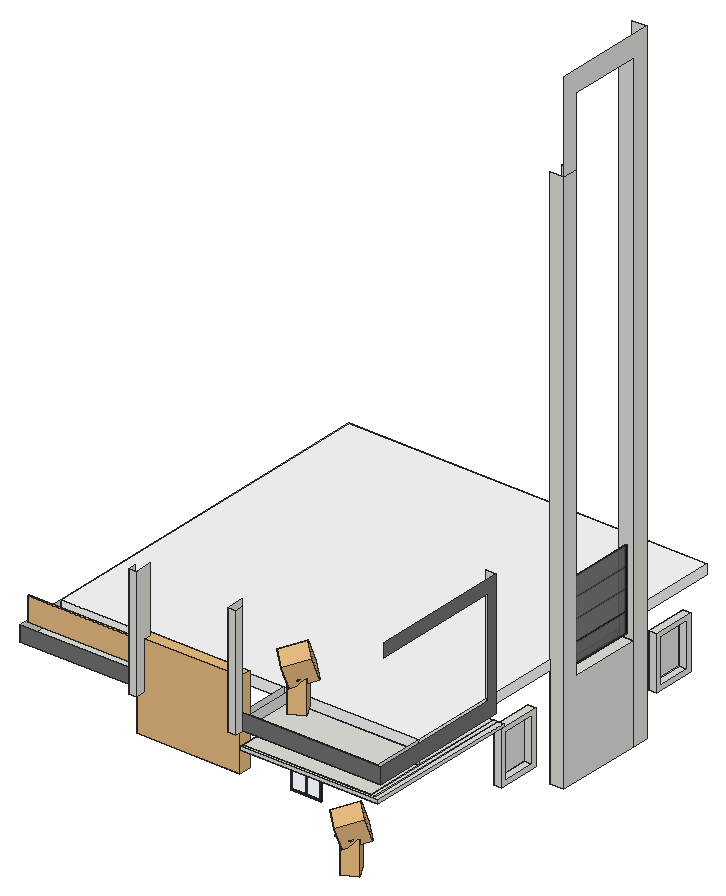
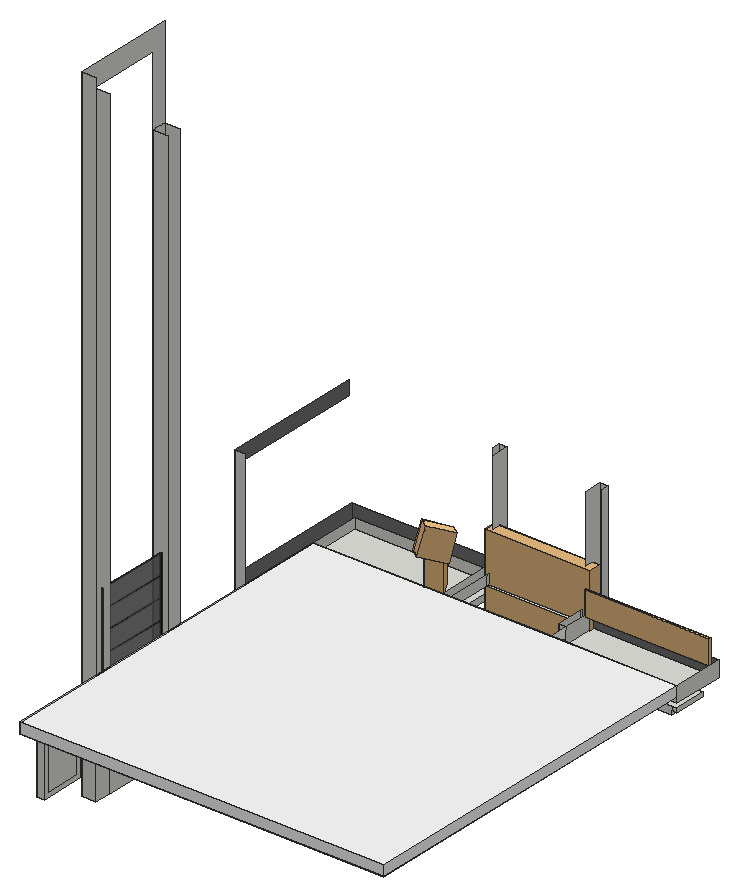
# SketchUp Ruby script. Lengths in inches.
U = 1.inch
M = Sketchup.active_model
def pt(a) = Geom::Point3d.new(a.map { |v| v * U })
def face(e, loops, mat)
  f = e.add_face(loops[0].map { |a| pt(a) })
  loops[1..].each { |l| e.add_face(l.map { |a| pt(a) }).erase! }
  f.material = f.back_material = mat if mat
  f
end
# faces: each face lists its corners as indices into pts; further lists are holes
def faces(e, pts, list, mat = nil) = list.each { |f| face(e, (f[0].is_a?(Array) ? f : [f]).map { |l| l.map { |i| pts[i] } }, mat) }
# xy, xz, yz: faces in a plane at the given z, y or x. An outline is a flat list of corners, or four numbers for a rectangle; further outlines are holes
def ring(l) = l.size == 4 ? [[l[0], l[1]], [l[2], l[1]], [l[2], l[3]], [l[0], l[3]]] : l.each_slice(2).to_a
def flat(e, list, mat, &to3) = list.each { |f| face(e, (f[0].is_a?(Array) ? f : [f]).map { |l| ring(l).map { |u, v| to3.(u, v) } }, mat) }
def xy(e, z, list, mat = nil) = flat(e, list, mat) { |x, y| [x, y, z] }
def xz(e, y, list, mat = nil) = flat(e, list, mat) { |x, z| [x, y, z] }
def yz(e, x, list, mat = nil) = flat(e, list, mat) { |y, z| [x, y, z] }
def lines(e, pts, list) = list.each { |a, b| e.add_line(pt(pts[a]), pt(pts[b])) }
# prism: a flat outline (further loops are holes) pulled along v
def prism(e, loops, v, mat = nil)
  f = face(e, loops, mat); d = Geom::Vector3d.new(v.map { |x| x * U })
  f.pushpull(f.normal.samedirection?(d) ? d.length : -d.length)
end
def box(e, o, s, mat = nil) = prism(e, [[o, [o[0] + s[0], o[1], o[2]], [o[0] + s[0], o[1] + s[1], o[2]], [o[0], o[1] + s[1], o[2]]]], [0, 0, s[2]], mat)
def at(x, y, z, deg = 0) = Geom::Transformation.translation(pt([x, y, z])) * Geom::Transformation.rotation(ORIGIN, Z_AXIS, deg.degrees)
def axes(o, x, y, z) = Geom::Transformation.new([*x, 0, *y, 0, *z, 0, *pt(o).to_a, 1])
def part(name) = M.definitions.add(name)
# library, detail: a bought-in or finely detailed component or shape, given as its bounding box
def library(name, o, s) = part(name).tap { |d| box(d.entities, o, s) }
def detail(e, o, s) = box(e.add_group.entities, o, s)
def put(e, d, t, mat = nil) = e.add_instance(d, t).tap { |i| i.material = mat if mat }
def group(e, t, mat = nil) = e.add_group.tap { |g| g.transformation = t; g.material = mat if mat }.entities
root = M.entities
M.materials.add("Material__1").color = [51, 42, 44]
M.materials.add("Material__2").color = [97, 132, 37]
M.materials.add("[0136_Charcoal]").color = [35, 35, 35]
M.materials.add("[Color M00]").color = [255, 255, 255]
M.materials.add("[Color M05]").color = [114, 114, 114]
M.materials.add("[Translucent_Glass_Blue]").color = [68, 104, 165]
M.materials["[Translucent_Glass_Blue]"].alpha = 0.07
M.materials.add("[Translucent_Glass_Green_Dark]").color = [33, 68, 103]
M.materials["[Translucent_Glass_Green_Dark]"].alpha = 0.08
M.materials.add("{045efeae-c101-a24d-bd9b-6f5600100adb}").color = [102, 102, 102]
M.materials["{045efeae-c101-a24d-bd9b-6f5600100adb}"].alpha = 0.7
M.materials.add("{16756a1b-d383-d94f-ad82-104813d2624f}").color = [19, 21, 27]
c1 = library("\#1",[-138.85,-135.75,0],[277.7,270.97,9.64])
c2 = library("\#2",[-34.84,-73.35,-33.91],[69.68,146.26,68.31])
c3 = library("\#5",[-4127.85,-1300.75,-2324.72],[5349.84,4521.24,5423.31])
c4 = part("\#3")
put(c4.entities,c3,at(450.18,-1111.4375,0),"Material__2")
c5 = part("12")
put(c5.entities,c1,axes([-49.79,-36.9375,349.64],[0.59279,0,0],[0,0.59279,0],[0,0,0.59279]),"Material__1")
put(c5.entities,c2,axes([-39.24,-18.18,177.19],[1.20819,-2.09264,0],[0,0,2.41638],[2.09264,1.20819,0]))
put(c5.entities,c4,axes([-83.44,-46.04,442.44],[-0.03636,-0.03293,-0.01473],[-0.00083,-0.02391,0.05549],[0.02997,-0.02791,-0.01158]))
c6 = part("Two-panel window \#1")
xy(c6.entities,-18,[[0,-31,2,35]],"[0136_Charcoal]")
xy(c6.entities,-16,[[0,-29,0.9375,33],[0.9375,-29,1.125,33],[1.125,-29,2,1],[1.125,3,2,33]],"[0136_Charcoal]")
xy(c6.entities,76,[[0,-29,0.9375,33],[0.9375,-29,1.125,33],[1.125,-29,2,1],[1.125,3,2,33]],"[0136_Charcoal]")
xy(c6.entities,78,[[0,-31,2,35]],"[0136_Charcoal]")
xz(c6.entities,-31,[[0,-18,2,78]],"[0136_Charcoal]")
xz(c6.entities,-29,[[0,-16,0.9375,76],[0.9375,-16,1.125,76],[1.125,-16,2,76]],"[0136_Charcoal]")
xz(c6.entities,1,[[1.125,-16,2,76]],"[0136_Charcoal]")
xz(c6.entities,3,[[1.125,-16,2,76]],"[0136_Charcoal]")
xz(c6.entities,33,[[0,-16,0.9375,76],[0.9375,-16,1.125,76],[1.125,-16,2,76]],"[0136_Charcoal]")
xz(c6.entities,35,[[0,-18,2,78]],"[0136_Charcoal]")
yz(c6.entities,0,[[[-31,-18,35,78],[-29,-16,33,76]]],"[0136_Charcoal]")
yz(c6.entities,0.9375,[[-29,-16,33,76]],"[Translucent_Glass_Blue]")
yz(c6.entities,1.125,[[1,-16,3,76]],"[0136_Charcoal]")
yz(c6.entities,1.125,[[-29,-16,1,76],[3,-16,33,76]],"[Translucent_Glass_Green_Dark]")
yz(c6.entities,2,[[[-31,-18,35,78],[-29,-16,1,76],[3,-16,33,76]]],"[0136_Charcoal]")
c7 = part("Two-panel window")
put(c7.entities,c6,axes([-31.84,50.72,0],[1,0,0],[0,1.1,0],[0,0,1]))
c8 = part("normal window")
put(c8.entities,c7,axes([114.26,44.3125,18],[0,1,0],[-0.90909,0,0],[0,0,1]))
c9 = part("Group\#20")
xy(c9.entities,0,[[[0,0,50.8125,62.9375],[5.49,5.49,45.32,57.45]],[5.49,5.49,45.32,57.45]])
xy(c9.entities,9.5625,[[[0,0,50.8125,62.9375],[5.49,5.49,45.32,57.45]]])
xz(c9.entities,0,[[0,0,50.8125,9.5625]])
xz(c9.entities,5.49,[[5.49,0,45.32,9.5625]])
xz(c9.entities,57.45,[[5.49,0,45.32,9.5625]])
xz(c9.entities,62.9375,[[0,0,50.8125,9.5625]])
yz(c9.entities,0,[[0,0,62.9375,9.5625]])
yz(c9.entities,5.49,[[5.49,0,57.45,9.5625]])
yz(c9.entities,45.32,[[5.49,0,57.45,9.5625]])
yz(c9.entities,50.8125,[[0,0,62.9375,9.5625]])
c10 = library("Facade Louver",[-2.17,-1,-2.17],[122.45,14.39,102.76])
c11 = part("Group\#29")
xy(c11.entities,-4.5625,[[0,-81.875,145.875,0]])
xy(c11.entities,0.59,[[-6.375,-89.375,-6.375,0,0,0,0,-81.875,145.875,-81.875,145.875,-89.375]])
xy(c11.entities,5.73,[[-6.375,-89.375,145.875,0]])
xz(c11.entities,-89.375,[[-6.375,0.59,145.875,5.73]])
xz(c11.entities,-81.875,[[0,-4.5625,145.875,0.59]])
xz(c11.entities,0,[[0,-4.5625,145.875,5.73],[-6.375,0.59,0,5.73]])
yz(c11.entities,-6.375,[[-89.375,0.59,0,5.73]])
yz(c11.entities,0,[[-81.875,-4.5625,0,0.59]])
yz(c11.entities,145.875,[[-81.875,-4.5625,0,-4.5625,0,5.73,-89.375,5.73,-89.375,0.59,-81.875,0.59]])
c12 = part("Furniture_0DcpanrIvuI8n_9Ae92L5A")
g1 = group(c12.entities,at(0,0,0))
box(g1,[-19.29,-0.2,0.39],[38.58,0.4,83.86],"{045efeae-c101-a24d-bd9b-6f5600100adb}")
g2 = group(c12.entities,at(0,0,0))
box(g2,[-19.68,-0.59,63.39],[39.36,1.18,0.39],"{16756a1b-d383-d94f-ad82-104813d2624f}")
box(g2,[-19.68,-0.59,42.52],[39.36,1.18,0.39],"{16756a1b-d383-d94f-ad82-104813d2624f}")
box(g2,[-19.68,-0.59,21.26],[39.36,1.18,0.39],"{16756a1b-d383-d94f-ad82-104813d2624f}")
xy(g2,0,[[-19.68,-0.59,19.68,0.59]],"{16756a1b-d383-d94f-ad82-104813d2624f}")
xy(g2,0.39,[[-19.68,-0.59,-19.29,0.59],[-19.68,-0.59,19.68,0.59],[19.29,-0.59,19.68,0.59]],"{16756a1b-d383-d94f-ad82-104813d2624f}")
xy(g2,84.25,[[-19.68,-0.59,19.68,0.59]],"{16756a1b-d383-d94f-ad82-104813d2624f}")
xy(g2,84.65,[[-19.68,-0.59,-19.29,0.59],[-19.68,-0.59,19.68,0.59],[19.29,-0.59,19.68,0.59]],"{16756a1b-d383-d94f-ad82-104813d2624f}")
xz(g2,-0.59,[[-19.68,0,19.68,0.39],[-19.68,0.39,-19.29,84.65],[19.29,0.39,19.68,84.65],[-19.68,84.25,19.68,84.65]],"{16756a1b-d383-d94f-ad82-104813d2624f}")
xz(g2,0.59,[[-19.68,0,19.68,0.39],[-19.68,0.39,-19.29,84.65],[19.29,0.39,19.68,84.65],[-19.68,84.25,19.68,84.65]],"{16756a1b-d383-d94f-ad82-104813d2624f}")
yz(g2,-19.68,[[-0.59,0,0.59,0.39],[-0.59,0.39,0.59,84.65],[-0.59,84.25,0.59,84.65]],"{16756a1b-d383-d94f-ad82-104813d2624f}")
yz(g2,-19.29,[[-0.59,0.39,0.59,84.65]],"{16756a1b-d383-d94f-ad82-104813d2624f}")
yz(g2,19.29,[[-0.59,0.39,0.59,84.65]],"{16756a1b-d383-d94f-ad82-104813d2624f}")
yz(g2,19.68,[[-0.59,0,0.59,0.39],[-0.59,0.39,0.59,84.65],[-0.59,84.25,0.59,84.65]],"{16756a1b-d383-d94f-ad82-104813d2624f}")
c13 = part("Glass Window")
put(c13.entities,c12,at(0,0,-42.32))
c14 = library("Glass Railings(black Handrails)",[-57.04,-132.55,0],[169.29,2.52,28.17])
xy(root,0.75,[[468.38,469.33,485.45,488.7]])
xy(root,0.8125,[[468.38,367.14,485.45,469.33]])
xy(root,101.63,[[317.76,98.82,317.76,103.01,468.38,103.01,468.38,283.99,480.13,283.99,480.13,98.82]])
xy(root,105.14,[[317.76,98.82,480.13,98.82,480.13,283.99,468.38,283.99,468.38,103.01,317.76,103.01]])
xy(root,113.12,[[468.38,384.58,485.45,469.33]])
xy(root,113.75,[[45.88,113.44,191.76,173.57]])
xy(root,120,[[317.76,103.01,317.76,113.44,468.38,113.44,468.38,273.38,480.01,273.38,480.01,103.01],[200.76,112.2,308.76,121.2],[317.76,113.44,468.38,173.57],[191.76,151.89,200.76,151.89,200.76,182.57,83.76,182.57,83.76,442.69,425.76,442.69,425.76,182.57,308.76,182.57,308.76,173.57,468.38,173.57,468.38,598.82,45.88,598.82,45.88,173.57,191.76,173.57]])
xz(root,91.69,[[191.76,120,200.76,252],[308.76,120,317.76,252]])
xz(root,98.82,[[317.76,101.63,480.13,105.14]])
xz(root,103.01,[[317.76,101.63,468.38,105.14]])
xz(root,103.01,[[317.76,120,480.01,138.375]],"[Color M05]")
xz(root,112.2,[[200.76,120,308.76,132]])
xz(root,113.44,[[317.76,120,468.38,132]])
xz(root,113.44,[[45.88,113.75,191.76,132]],"[Color M05]")
xz(root,151.89,[[191.76,120,200.76,132]])
xz(root,173.57,[[317.76,105.14,468.38,120],[45.88,113.75,191.76,120],[308.76,120,317.76,132]])
xz(root,273.38,[[468.38,120,480.01,268.25]])
xz(root,283.99,[[468.38,101.63,480.13,105.14]])
xz(root,367.14,[[468.38,0.8125,485.45,648]])
xz(root,384.58,[[468.38,113.12,485.45,648]])
xz(root,469.33,[[468.38,0.75,485.45,0.8125],[468.38,0.8125,485.45,113.12],[468.38,113.12,485.45,729.3125]])
xz(root,488.7,[[468.38,0.75,485.45,754.625]])
yz(root,45.88,[[113.44,113.75,173.57,132]])
yz(root,191.76,[[113.44,113.75,151.89,132],[151.89,113.75,173.57,120],[91.69,120,100.69,252]])
yz(root,200.76,[[91.69,120,112.2,252],[112.2,120,121.2,132],[121.2,120,151.89,132]])
yz(root,308.76,[[91.69,120,112.2,252],[112.2,120,121.2,132],[121.2,120,173.57,132]])
yz(root,317.76,[[98.82,101.63,100.69,105.14],[100.69,101.63,103.01,105.14],[91.69,120,100.69,252],[113.44,120,173.57,132]])
yz(root,468.38,[[469.33,0.75,488.7,58.375],[367.14,0.8125,469.33,0.8125,469.33,113.12,384.58,113.12,384.58,120,367.14,120],[469.33,58.375,488.7,120],[103.01,101.63,173.57,105.14],[173.57,101.63,283.99,105.14],
  [384.58,113.12,469.33,120],[113.44,120,273.38,132],[367.14,120,384.58,132],[469.33,120,488.7,132]])
yz(root,480.01,[[103.01,120,273.38,120,273.38,268.25,107.51,268.25,107.51,252,261.76,252,261.76,138.375,103.01,138.375]],"[Color M05]")
yz(root,480.13,[[98.82,101.63,283.99,105.14]])
yz(root,485.45,[[469.33,0.75,488.7,0.75,488.7,754.625,367.14,754.625,367.14,648,384.58,648,384.58,729.3125,469.33,729.3125],[367.14,0.8125,469.33,0.8125,469.33,113.12,384.58,113.12,384.58,648,367.14,648]])
put(root,c5,axes([434.27,124.18,2.65],[0.1092,0,0],[0,0.1092,0],[0,0,0.1092]))
put(root,c8,axes([299.72,167.1875,26.47],[0.5481,0,0],[0,0.441,0],[0,0,0.63]))
put(root,c9,axes([468.38,283.99,35.83],[0,1,0],[0,0,1],[1,0,0]))
put(root,c9,axes([468.38,512.67,35.83],[0,1,0],[0,0,1],[1,0,0]))
put(root,c10,at(193.59,104.35,75.19))
g3 = group(root,at(317.76,173.57,98.13))
box(g3,[0,-70.5625,0],[155.875,180.3125,7.01])
put(root,c11,axes([52.26,173.57,103.24],[1,0,0],[0,0.42,0],[0,0,1]))
put(root,c13,axes([476.49,426.95,164.48],[0,-2.15265,0],[1,0,0],[0,0,1.1124]))
g4 = group(root,at(74.76,451.69,120),"[Color M00]")
xy(g4,0,[[-28.875,-278.125,393.625,147.125]])
xy(g4,12,[[-28.875,-278.125,393.625,147.125]])
xz(g4,-278.125,[[-28.875,0,117,12],[117,0,393.625,12]])
xz(g4,147.125,[[-28.875,0,393.625,12]])
yz(g4,-28.875,[[-278.125,0,147.125,12]])
yz(g4,117,[[-299.81,0,-278.125,12]])
yz(g4,393.625,[[-278.125,0,147.125,12]])
put(root,c5,axes([342.25,161.12,124.06],[0.1092,0,0],[0,0.1092,0],[0,0,0.1092]))
put(root,c14,axes([96.01,255.35,130.91],[0.85302,0,0],[0,1,0],[0,0,1]))
